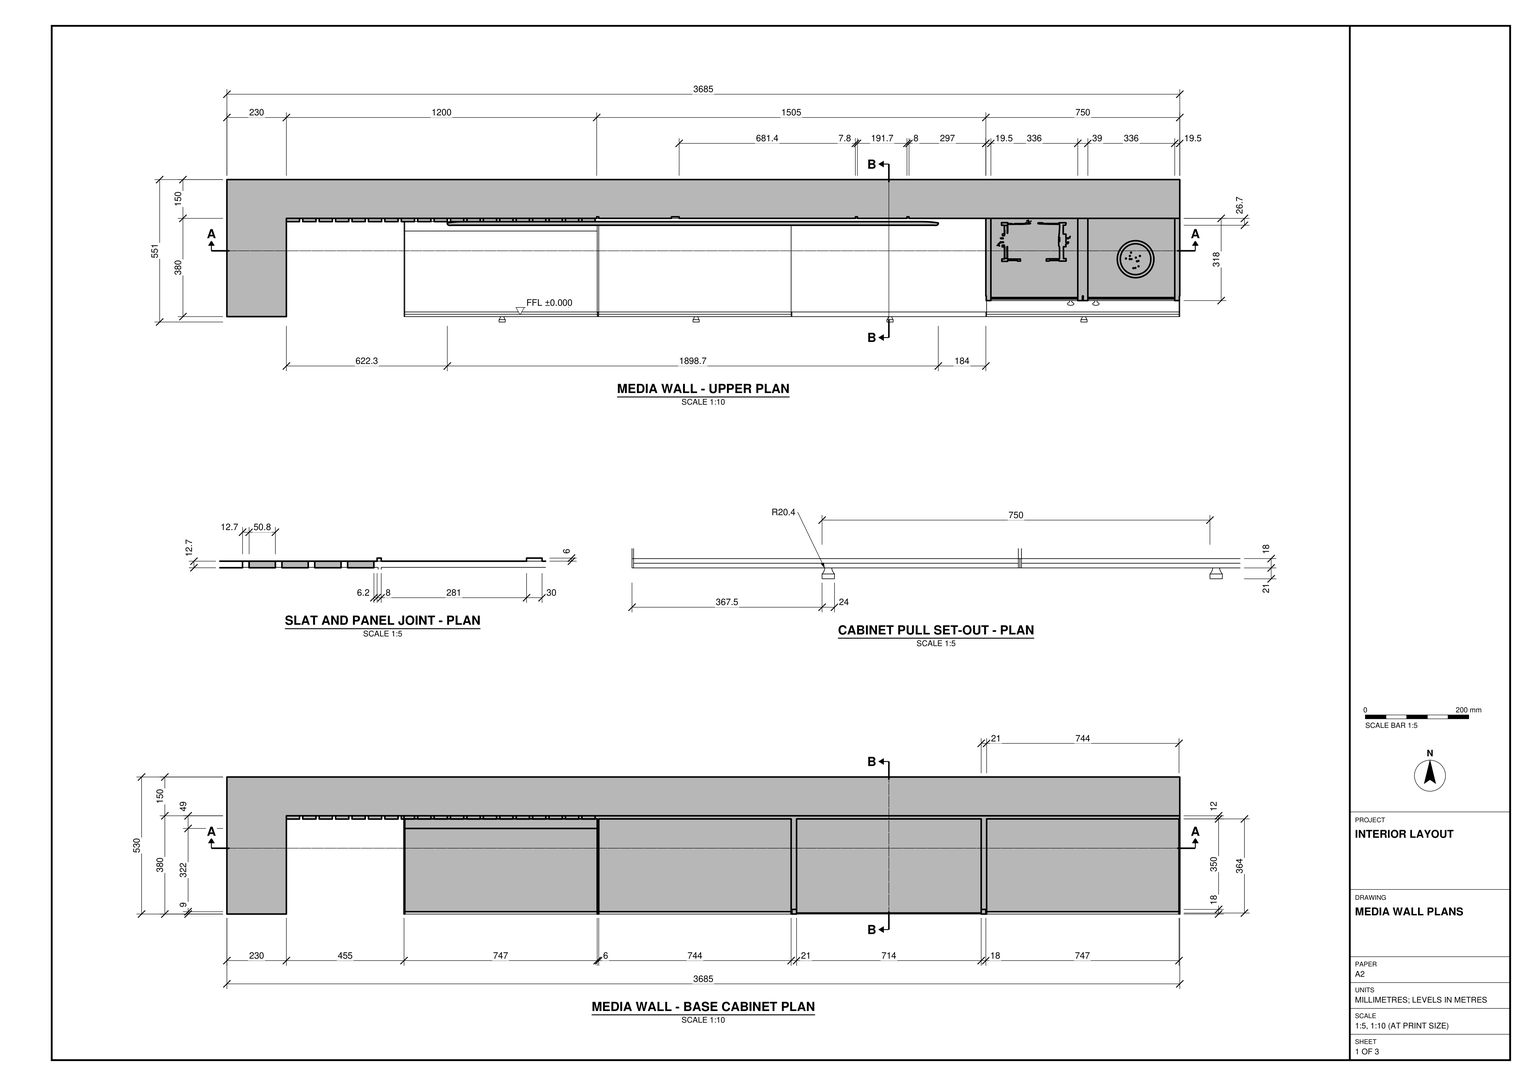
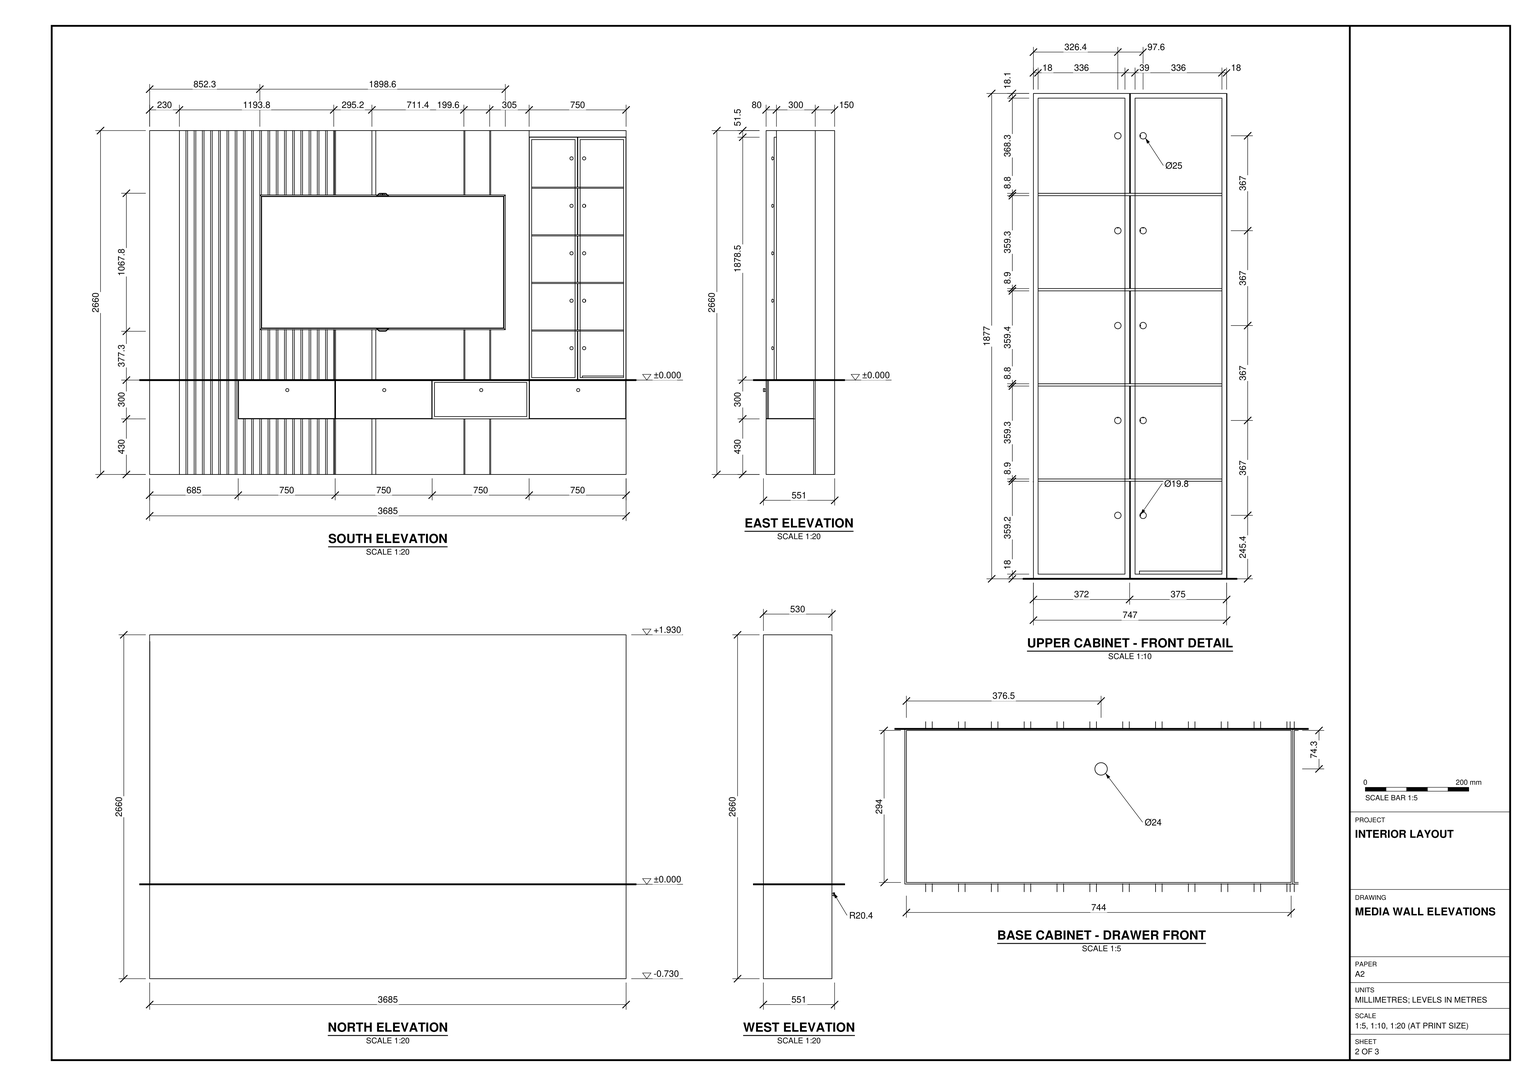
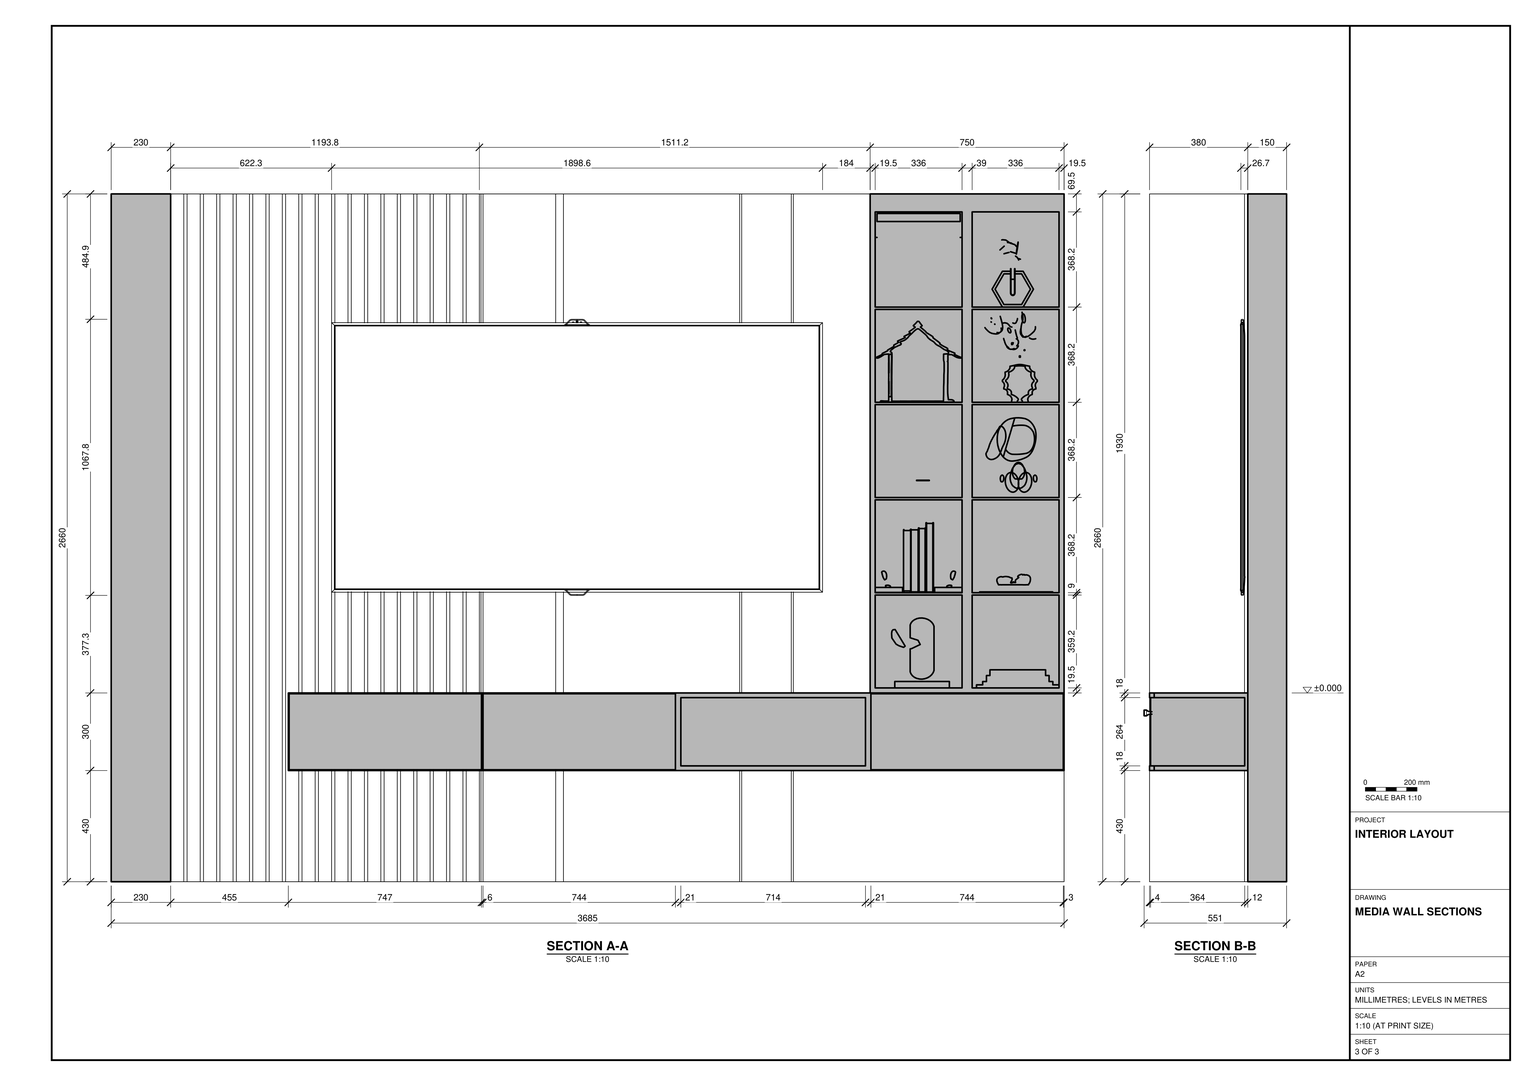
Build the media wall in SketchUp from task_files/diagram_01.pdf. Work in millimetres. The complete assembly, including the projecting cabinet pulls, is 3685 mm wide, 551 mm deep and 2660 mm high. Use the 0 mm datum shown at the top of the base cabinets: the wall extends from −730 mm to 1930 mm relative to that datum.

Use the plans to form the 150 mm thick backing wall and its left return. Facing the wall as in the south elevation, start the vertical slats immediately to the right of the return. Continue with flat panels, following the joint positions in the drawings. Place the screen across the transition from slats to panels. Below it, model the floating run of four base cabinet bays, including the drawer fronts, inset front detail and projecting pulls. Leave the wall face visible beneath the run.

At the right end, model the upper display cabinet with its centre divider, aligned shelves, framed fronts and pulls. Place books and loose display objects on the shelves as shown; any suitable library components may be used for these items. Keep the wall and each joinery piece in separate groups or components, and use components for repeated parts such as slats and pulls. Save one SketchUp model as output_files/media_wall_with_floating_cabinets_and_display_shelves.skp.

# SketchUp Ruby script. Lengths in millimetres.
U = 1.mm
M = Sketchup.active_model
def pt(a) = Geom::Point3d.new(a.map { |v| v * U })
def face(e, loops, mat)
  f = e.add_face(loops[0].map { |a| pt(a) })
  loops[1..].each { |l| e.add_face(l.map { |a| pt(a) }).erase! }
  f.material = f.back_material = mat if mat
  f
end
# faces: each face lists its corners as indices into pts; further lists are holes
def faces(e, pts, list, mat = nil) = list.each { |f| face(e, (f[0].is_a?(Array) ? f : [f]).map { |l| l.map { |i| pts[i] } }, mat) }
# xy, xz, yz: faces in a plane at the given z, y or x. An outline is a flat list of corners, or four numbers for a rectangle; further outlines are holes
def ring(l) = l.size == 4 ? [[l[0], l[1]], [l[2], l[1]], [l[2], l[3]], [l[0], l[3]]] : l.each_slice(2).to_a
def flat(e, list, mat, &to3) = list.each { |f| face(e, (f[0].is_a?(Array) ? f : [f]).map { |l| ring(l).map { |u, v| to3.(u, v) } }, mat) }
def xy(e, z, list, mat = nil) = flat(e, list, mat) { |x, y| [x, y, z] }
def xz(e, y, list, mat = nil) = flat(e, list, mat) { |x, z| [x, y, z] }
def yz(e, x, list, mat = nil) = flat(e, list, mat) { |y, z| [x, y, z] }
def lines(e, pts, list) = list.each { |a, b| e.add_line(pt(pts[a]), pt(pts[b])) }
# prism: a flat outline (further loops are holes) pulled along v
def prism(e, loops, v, mat = nil)
  f = face(e, loops, mat); d = Geom::Vector3d.new(v.map { |x| x * U })
  f.pushpull(f.normal.samedirection?(d) ? d.length : -d.length)
end
def box(e, o, s, mat = nil) = prism(e, [[o, [o[0] + s[0], o[1], o[2]], [o[0] + s[0], o[1] + s[1], o[2]], [o[0], o[1] + s[1], o[2]]]], [0, 0, s[2]], mat)
def at(x, y, z, deg = 0) = Geom::Transformation.translation(pt([x, y, z])) * Geom::Transformation.rotation(ORIGIN, Z_AXIS, deg.degrees)
def axes(o, x, y, z) = Geom::Transformation.new([*x, 0, *y, 0, *z, 0, *pt(o).to_a, 1])
def part(name) = M.definitions.add(name)
# library, detail: a bought-in or finely detailed component or shape, given as its bounding box
def library(name, o, s) = part(name).tap { |d| box(d.entities, o, s) }
def detail(e, o, s) = box(e.add_group.entities, o, s)
def put(e, d, t, mat = nil) = e.add_instance(d, t).tap { |i| i.material = mat if mat }
def group(e, t, mat = nil) = e.add_group.tap { |g| g.transformation = t; g.material = mat if mat }.entities
root = M.entities
M.materials.add("E04_Green_Bloom").color = [255, 255, 49]
M.materials.add("Plastic_Metalic_Black").color = [8, 8, 8]
M.materials.add("[Carpet Berber Multi]").color = [151, 134, 122]
M.materials.add("[Granite Dark Gray]").color = [69, 68, 68]
M.materials.add("[Metal Steel Textured]").color = [106, 110, 123]
M.materials.add("[Resin Turquoise]").color = [117, 218, 223]
M.materials.add("[Stone_Granite_Midnite]").color = [98, 95, 96]
M.materials.add("[Stone_Masonry_Multi]").color = [182, 175, 164]
M.materials.add("[Stone_Pavers_Flagstone_Gray]").color = [162, 162, 162]
M.materials.add("[Translucent Glass Blue]").color = [100, 149, 237]
M.materials["[Translucent Glass Blue]"].alpha = 0.5
M.materials.add("[Translucent Glass Dark Green]").color = [62, 91, 5]
M.materials["[Translucent Glass Dark Green]"].alpha = 0.5
M.materials.add("[Translucent Glass Tinted]").color = [8, 201, 241]
M.materials["[Translucent Glass Tinted]"].alpha = 0.5
M.materials.add("[Water Pool Light]").color = [64, 149, 167]
M.materials["[Water Pool Light]"].alpha = 0.6
M.materials.add("[Wood Bamboo]").color = [177, 105, 43]
M.materials.add("[Wood Floor Parquet]").color = [145, 89, 39]
M.materials.add("[Wood Veneer 01]").color = [120, 70, 37]
M.materials.add("[Wood Veneer 02]").color = [190, 128, 91]
c1 = part("Fluted wall panel")
box(c1.entities,[0,0,0],[50.8,12.7,2660])
box(c1.entities,[63.5,0,0],[50.8,12.7,2660])
box(c1.entities,[127,0,0],[50.8,12.7,2660])
box(c1.entities,[190.5,0,0],[50.8,12.7,2660])
box(c1.entities,[254,0,0],[50.8,12.7,2660])
box(c1.entities,[317.5,0,0],[50.8,12.7,2660])
box(c1.entities,[381,0,0],[50.8,12.7,2660])
box(c1.entities,[444.5,0,0],[50.8,12.7,2660])
box(c1.entities,[508,0,0],[50.8,12.7,2660])
box(c1.entities,[571.5,0,0],[50.8,12.7,2660])
box(c1.entities,[635,0,0],[50.8,12.7,2660])
box(c1.entities,[698.5,0,0],[50.8,12.7,2660])
box(c1.entities,[762,0,0],[50.8,12.7,2660])
box(c1.entities,[825.5,0,0],[50.8,12.7,2660])
box(c1.entities,[889,0,0],[50.8,12.7,2660])
box(c1.entities,[952.5,0,0],[50.8,12.7,2660])
box(c1.entities,[1016,0,0],[50.8,12.7,2660])
box(c1.entities,[1143,0,0],[50.8,12.7,2660])
xy(c1.entities,0,[[1079.5,0,1130.3,12.7]])
xy(c1.entities,2660,[[1079.5,0,1130.3,12.7]])
xz(c1.entities,0,[[1079.5,0,1130.3,2660]],"[Wood Floor Parquet]")
xz(c1.entities,12.7,[[1079.5,0,1130.3,2660]])
yz(c1.entities,1079.5,[[0,0,12.7,2660]])
yz(c1.entities,1130.3,[[0,0,12.7,2660]])
c2 = library("download?mid=50c7180b9fccec56d493bfe20f94b6ab&ctyp=sp&cv=p8.",[3795.5,1113.3,453.6],[1898.6,14.5,1067.8])
c3 = part("photo frame")
g1 = group(c3.entities,at(3094.9,8.6,0.8))
g2 = group(g1,at(0,0,0))
yz(g2,0,[[12.1,-0.8,0,0,33.6,534.4,45.7,533.6]],"Plastic_Metalic_Black")
yz(g2,8.6,[[7,8.2,39.5,525.3,33.1,525.8,0.5,8.6]],"Plastic_Metalic_Black")
yz(g2,393.2,[[7,8.2,0.5,8.6,33.1,525.8,39.5,525.3]],"Plastic_Metalic_Black")
yz(g2,401.8,[[12.1,-0.8,45.7,533.6,33.6,534.4,0,0]],"Plastic_Metalic_Black")
p = [[0,12.1,-0.8],[401.8,12.1,-0.8],[401.8,0,0],[0,0,0],[401.8,45.7,533.6],[0,45.7,533.6],
  [8.6,12.6,7.9],[393.2,12.6,7.9],[393.2,45.1,525],[8.6,45.1,525],[401.8,33.6,534.4],[0,33.6,534.4],
  [393.2,0.5,8.6],[8.6,0.5,8.6],[8.6,33.1,525.8],[393.2,33.1,525.8],[393.2,7,8.2],[8.6,7,8.2],
  [393.2,39.5,525.3],[8.6,39.5,525.3],[358.7,9.2,42.7],[43.2,9.2,42.7],[43.2,37.4,490.9],[358.7,37.4,490.9]]
faces(g2,p,[[0,1,2,3],[[4,1,0,5],[6,7,8,9]],[[2,10,11,3],[12,13,14,15]],[16,17,13,12],[19,18,15,14],[4,5,11,10]],"Plastic_Metalic_Black")
faces(g2,p,[[[17,16,18,19],[20,21,22,23]],[21,20,23,22]])
lines(g2,p,[[6,17],[9,19],[8,18],[7,16]])
c4 = library("Hexagonal flower vase",[-26.2,-52.8,0],[186.2,162.5,287.3])
c5 = library("Hexagonal flower vase \#1",[-6.8,-48.8,-5.9],[192.1,162.5,293.2])
c6 = library("Miniature+Toy+House+–+Teal+Roof,+Yellow+Trim,+and+Heart-Shap",[-518,0,0],[1389.1,735.6,998.2])
c7 = library("Copper+Vase+W.+Flowers",[-61.6,-66.4,0],[634.8,593.9,639.8])
c8 = library("Children's+Sailboat+Wall+Shelf++Decorative+Nursery+Bookcase+",[77.4,0,793.6],[1200,350,1226.4])
c9 = library("cheburashka",[1021,1096.6,-13.6],[484.8,208,352.2])
c10 = library("APARADOR+DE+LIVROS+CACHORRO",[2417,259.3,62.1],[359.3,219.7,270.8])
c11 = library("Buddha Fountain",[-19.2,-33.2,-3.3],[3019.4,1766,2624.3])
c12 = library("HORSE",[1857.3,-2493,-0.9],[2418.1,1518.6,2900.9])
c13 = library("16-POIGNEE CLC2",[-12.8,-12.5,0],[25,25,25])
c14 = library("14-POIGNEE CLC2",[-12,-12,0],[24,24,30])
c15 = library("Grupo\#181",[-9.6,-14,0],[182,201.9,289.1])
xy(root,0,[[0,0,230,530],[230,380,3685,530]])
xy(root,430,[[685,0,1435,18]])
xy(root,430,[[685,18,3685,380]],"[Carpet Berber Multi]")
xy(root,430,[[1435,0,2185,18],[2185,0,2935,18],[2935,0,3685,18]],"[Metal Steel Textured]")
xy(root,433,[[688,9,1432,18],[1438,9,2182,18],[2938,9,3682,18],[688,18,1432,368],[1438,18,2182,368],
  [2938,18,3682,368]],"[Carpet Berber Multi]")
xy(root,433,[[688,0,1432,9],[1438,0,2182,9],[2938,0,3682,9]],"[Metal Steel Textured]")
xy(root,448,[[2203,4,2917,18],[2203,18,2917,368]],"[Carpet Berber Multi]")
xy(root,448,[[2203,0,2917,4]],"[Metal Steel Textured]")
xy(root,712,[[2203,4,2917,18],[2203,18,2917,368]],"[Carpet Berber Multi]")
xy(root,712,[[2203,0,2917,4]],"[Metal Steel Textured]")
xy(root,727,[[688,9,1432,18],[1438,9,2182,18],[2938,9,3682,18],[688,18,1432,368],[1438,18,2182,368],
  [2938,18,3682,368]],"[Carpet Berber Multi]")
xy(root,727,[[688,0,1432,9],[1438,0,2182,9],[2938,0,3682,9]],"[Metal Steel Textured]")
xy(root,730,[[1430,380,1438,386],[1719,380,1749,386],[2430.4,380,2438.3,386],[2630,380,2638,386]])
xy(root,730,[[685,18,3685,18,3685,80,2935,80,2935,380,685,380]],"[Carpet Berber Multi]")
xy(root,730,[[685,0,1435,18],[1435,0,2185,18],[2185,0,2935,18],[2935,0,3685,18]],"[Metal Steel Textured]")
xy(root,730,[[2935,80,3685,380]],"[Wood Veneer 01]")
xy(root,731.5,[[2936.5,62,3308.5,80],[3308.5,62,3310,80],[3310,62,3311.5,80],[3311.5,62,3683.5,80]],"[Wood Veneer 01]")
xy(root,749.5,[[3346.4,68.5,3665.5,73.5]])
xy(root,749.5,[[2954.5,62,3290.5,68.5],[3329.5,62,3665.5,68.5]],"[Metal Steel Textured]")
xy(root,749.5,[[2954.5,68.5,3290.5,73.5],[3329.5,68.5,3346.4,73.5]],"[Translucent Glass Tinted]")
xy(root,749.5,[[2954.5,73.5,3290.5,380],[3329.5,73.5,3346.4,73.5,3346.4,331.9,3665.5,331.9,3665.5,380,3329.5,380],[3346.4,73.5,3665.5,331.9]],"[Wood Veneer 01]")
xy(root,761.4,[[[3346.4,73.5,3665.5,331.9],[3370.3,92.8,3641.6,301.1]]],"[Stone_Masonry_Multi]")
xy(root,774.1,[[[3370.3,92.8,3641.6,301.1],[3384.9,111.7,3627,282.3]]],"[Stone_Masonry_Multi]")
xy(root,797.4,[[[3384.9,111.7,3627,282.3],[3398.3,130,3613.6,264.9]]],"[Stone_Masonry_Multi]")
xy(root,819.6,[[[3398.3,130,3613.6,264.9],[3424.8,156.6,3598.4,238.2]]],"[Stone_Masonry_Multi]")
xy(root,926.4,[[3424.8,156.6,3598.4,238.2]],"[Stone_Pavers_Flagstone_Gray]")
xy(root,1108.7,[[2954.5,62,3290.5,80],[3290.5,62,3308.5,80],[3308.5,62,3310,80],[3310,62,3311.5,80],[3311.5,62,3329.5,80],
  [3329.5,62,3665.5,80],[2954.5,80,3290.5,380],[3329.5,80,3665.5,380]],"[Wood Veneer 01]")
xy(root,1117.5,[[2954.5,68.5,3290.5,73.5],[3329.5,68.5,3665.5,73.5]],"[Translucent Glass Tinted]")
xy(root,1117.7,[[2954.5,68.5,3290.5,73.5],[3329.5,68.5,3665.5,73.5]],"[Translucent Glass Tinted]")
xy(root,1117.7,[[2954.5,62,3290.5,68.5],[3290.5,62,3308.5,80],[3308.5,62,3310,80],[3310,62,3311.5,80],[3311.5,62,3329.5,80],
  [3329.5,62,3665.5,68.5],[2954.5,73.5,3290.5,380],[3329.5,73.5,3665.5,380]],"[Wood Veneer 01]")
xy(root,1476.9,[[2954.5,62,3290.5,380],[3290.5,62,3308.5,80],[3308.5,62,3310,80],[3310,62,3311.5,80],[3311.5,62,3329.5,80],
  [3329.5,62,3665.5,380]],"[Wood Veneer 01]")
xy(root,1485.7,[[2954.5,68.5,3290.5,73.5],[3329.5,68.5,3665.5,73.5]],"[Translucent Glass Tinted]")
xy(root,1485.9,[[2954.5,62,3290.5,68.5],[3329.5,62,3665.5,68.5]],"[Metal Steel Textured]")
xy(root,1485.9,[[2954.5,68.5,3290.5,73.5],[3329.5,68.5,3665.5,73.5]],"[Translucent Glass Tinted]")
xy(root,1485.9,[[3290.5,62,3308.5,80],[3308.5,62,3310,80],[3310,62,3311.5,80],[3311.5,62,3329.5,80],[2954.5,73.5,3290.5,380],
  [3329.5,73.5,3665.5,380]],"[Wood Veneer 01]")
xy(root,1845.1,[[2954.5,62,3290.5,380],[3290.5,62,3308.5,80],[3308.5,62,3310,80],[3310,62,3311.5,80],[3311.5,62,3329.5,80],
  [3329.5,62,3665.5,80],[3329.5,80,3665.5,380]],"[Wood Veneer 01]")
xy(root,1853.9,[[2954.5,68.5,3290.5,73.5],[3329.5,68.5,3665.5,73.5]],"[Translucent Glass Tinted]")
xy(root,1854.1,[[3329.5,62,3665.5,68.5]],"[Metal Steel Textured]")
xy(root,1854.1,[[2954.5,68.5,3290.5,73.5],[3329.5,68.5,3665.5,73.5]],"[Translucent Glass Tinted]")
xy(root,1854.1,[[2954.5,62,3290.5,68.5],[3290.5,62,3308.5,80],[3308.5,62,3310,80],[3310,62,3311.5,80],[3311.5,62,3329.5,80],
  [2954.5,73.5,3290.5,380],[3329.5,73.5,3665.5,380]],"[Wood Veneer 01]")
xy(root,2213.3,[[2954.5,62,3290.5,380],[3290.5,62,3308.5,80],[3308.5,62,3310,80],[3310,62,3311.5,80],[3311.5,62,3329.5,80],
  [3329.5,62,3665.5,380]],"[Wood Veneer 01]")
xy(root,2222.1,[[2954.5,68.5,3290.5,73.5],[3329.5,68.5,3665.5,73.5]],"[Translucent Glass Tinted]")
xy(root,2222.3,[[2954.5,62,3290.5,68.5],[3329.5,62,3665.5,68.5]],"[Metal Steel Textured]")
xy(root,2222.3,[[2954.5,68.5,3290.5,73.5],[3329.5,68.5,3665.5,73.5]],"[Translucent Glass Tinted]")
xy(root,2222.3,[[3290.5,62,3308.5,80],[3308.5,62,3310,80],[3310,62,3311.5,80],[3311.5,62,3329.5,80],[2954.5,73.5,3290.5,380],
  [3329.5,73.5,3665.5,380]],"[Wood Veneer 01]")
xy(root,2590.3,[[2954.5,68.5,3290.5,73.5],[3329.5,68.5,3665.5,73.5]],"[Translucent Glass Tinted]")
xy(root,2590.5,[[2954.5,62,3290.5,68.5],[3329.5,62,3665.5,68.5],[2954.5,68.5,3290.5,80],[3329.5,68.5,3665.5,80],[2954.5,80,3290.5,380],
  [3329.5,80,3665.5,380]],"[Wood Veneer 01]")
xy(root,2608.5,[[2936.5,62,3308.5,80],[3311.5,62,3683.5,80]],"[Metal Steel Textured]")
xy(root,2608.5,[[3308.5,62,3310,80],[3310,62,3311.5,80]],"[Wood Veneer 01]")
xy(root,2660,[[0,0,230,0,230,380,1430,380,1430,386,1438,386,1438,380,1719,380,1719,386,1749,386,1749,380,2430.4,380,2430.4,386,2438.3,386,2438.3,380,2630,380,2630,386,2638,386,2638,380,3685,380,3685,530,0,530]],"[Granite Dark Gray]")
xy(root,2660,[[2935,80,3685,380]],"[Wood Veneer 02]")
xz(root,0,[[0,0,230,2660]],"[Granite Dark Gray]")
xz(root,0,[[[685,430,1435,730],[688,433,1432,727]],[[1435,430,2185,730],[1438,433,2182,727]],[[2185,430,2935,730],[2203,448,2917,712]],[[2935,430,3685,730],[2938,433,3682,727]]],"[Metal Steel Textured]")
xz(root,4,[[2203,448,2917,712]],"[Translucent Glass Dark Green]")
xz(root,9,[[688,433,1432,727],[1438,433,2182,727],[2938,433,3682,727]],"[Translucent Glass Blue]")
xz(root,18,[[[685,430,1435,730],[688,433,1432,727]],[[1435,430,2185,730],[1438,433,2182,727]],[[2185,430,2935,730],[2203,448,2917,712]],[[2935,430,3685,730],[2938,433,3682,727]]])
xz(root,62,[[2936.5,731.5,3308.5,731.5,3308.5,1108.7,3290.5,1108.7,3290.5,749.5,2954.5,749.5,2954.5,2590.5,3290.5,2590.5,3290.5,2222.3,3308.5,2222.3,3308.5,2608.5,2936.5,2608.5],[3311.5,731.5,3683.5,731.5,3683.5,2608.5,3311.5,2608.5,3311.5,2222.3,3329.5,2222.3,3329.5,2590.5,3665.5,2590.5,3665.5,749.5,3329.5,749.5,3329.5,1108.7,3311.5,1108.7],[2954.5,1108.7,3665.5,1117.7],[3290.5,1117.7,3308.5,1476.9],[3311.5,1117.7,3329.5,1476.9],
  [2954.5,1476.9,3665.5,1485.9],[3290.5,1485.9,3308.5,1845.1],[3311.5,1485.9,3329.5,1845.1],[2954.5,1845.1,3665.5,1854.1],[3290.5,1854.1,3308.5,2213.3],
  [3311.5,1854.1,3329.5,2213.3],[2954.5,2213.3,3665.5,2222.3]],"[Metal Steel Textured]")
xz(root,62,[[3308.5,731.5,3310,1108.7],[3310,731.5,3311.5,1108.7],[3308.5,1117.7,3310,1476.9],[3310,1117.7,3311.5,1476.9],[3308.5,1485.9,3310,1845.1],
  [3310,1485.9,3311.5,1845.1],[3308.5,1854.1,3310,2213.3],[3310,1854.1,3311.5,2213.3],[3308.5,2222.3,3310,2608.5],[3310,2222.3,3311.5,2608.5]],"[Wood Veneer 01]")
xz(root,68.5,[[2954.5,749.5,3290.5,1117.5],[3329.5,749.5,3665.5,1117.5],[2954.5,1117.7,3290.5,1485.7],[3329.5,1117.7,3665.5,1485.7],[2954.5,1485.9,3290.5,1853.9],
  [3329.5,1485.9,3665.5,1853.9],[2954.5,1854.1,3290.5,2222.1],[3329.5,1854.1,3665.5,2222.1],[2954.5,2222.3,3290.5,2590.3],[3329.5,2222.3,3665.5,2590.3]],"[Translucent Glass Blue]")
xz(root,73.5,[[3346.4,749.5,3665.5,761.4]],"[Stone_Masonry_Multi]")
xz(root,73.5,[[2954.5,749.5,3290.5,1117.5],[3329.5,749.5,3329.5,1117.5,3665.5,1117.5,3665.5,761.4,3346.4,761.4,3346.4,749.5],[2954.5,1117.7,3290.5,1485.7],[3329.5,1117.7,3665.5,1485.7],[2954.5,1485.9,3290.5,1853.9],
  [3329.5,1485.9,3665.5,1853.9],[2954.5,1854.1,3290.5,2222.1],[3329.5,1854.1,3665.5,2222.1],[2954.5,2222.3,3290.5,2590.3],[3329.5,2222.3,3665.5,2590.3]],"[Translucent Glass Tinted]")
xz(root,80,[[[2935,730,3685,2610],[2936.5,731.5,3683.5,2608.5]],[3308.5,731.5,3310,1108.7],[3310,731.5,3311.5,1108.7],[3308.5,1117.7,3310,1476.9],[3310,1117.7,3311.5,1476.9],
  [3308.5,1485.9,3310,1845.1],[3310,1485.9,3311.5,1845.1],[3308.5,1854.1,3310,2213.3],[3310,1854.1,3311.5,2213.3],[3308.5,2222.3,3310,2608.5],
  [3310,2222.3,3311.5,2608.5]],"[Wood Veneer 01]")
xz(root,80,[[2935,2610,3685,2660]],"[Wood Veneer 02]")
xz(root,92.8,[[3370.3,761.4,3641.6,774.1]],"[Stone_Granite_Midnite]")
xz(root,111.7,[[3384.9,774.1,3627,797.4]],"[Stone_Granite_Midnite]")
xz(root,130,[[3398.3,797.4,3613.6,819.6]],"[Stone_Granite_Midnite]")
xz(root,156.6,[[3424.8,819.6,3598.4,926.4]],"[Stone_Pavers_Flagstone_Gray]")
xz(root,238.2,[[3424.8,819.6,3598.4,926.4]],"[Stone_Pavers_Flagstone_Gray]")
xz(root,264.9,[[3398.3,797.4,3613.6,819.6]],"[Stone_Granite_Midnite]")
xz(root,282.3,[[3384.9,774.1,3627,797.4]],"[Stone_Granite_Midnite]")
xz(root,301.1,[[3370.3,761.4,3641.6,774.1]],"[Stone_Granite_Midnite]")
xz(root,331.9,[[3346.4,749.5,3665.5,761.4]],"[Stone_Pavers_Flagstone_Gray]")
xz(root,368,[[688,433,1432,727]])
xz(root,368,[[1438,433,2182,727],[2938,433,3682,727],[2203,448,2917,712]],"[Carpet Berber Multi]")
xz(root,380,[[230,0,1430,0,1430,430,685,430,685,730,1430,730,1430,2660,230,2660],[1430,0,1438,430],[1438,0,1719,430],[1719,0,1749,430],[1749,0,2430.4,430],
  [2430.4,0,2438.3,430],[2438.3,0,2630,430],[2630,0,2638,430],[2638,0,3685,430],[1438,730,1719,2660],
  [1749,730,2430.4,2660],[2438.3,730,2630,2660],[2638,730,2935,2660]])
xz(root,380,[[2954.5,749.5,3290.5,1108.7],[3329.5,749.5,3665.5,1108.7],[2954.5,1126.7,3290.5,1476.9],[3329.5,1126.7,3665.5,1476.9],[3329.5,1494.9,3665.5,1845.1],
  [2954.5,1863.1,3290.5,2213.3],[3329.5,1863.1,3665.5,2213.3],[2954.5,2231.3,3290.5,2590.5],[3329.5,2231.3,3665.5,2590.5]],"[Water Pool Light]")
xz(root,380,[[685,430,1430,730],[1430,430,1438,730],[1438,430,1719,730],[1719,430,1749,730],[1749,430,2430.4,730],
  [2430.4,430,2438.3,730],[2438.3,430,2630,730],[2630,430,2638,730],[2638,430,3685,730],[[2935,730,3685,2660],[2954.5,2222.3,3290.5,2590.5],[3329.5,2222.3,3665.5,2590.5],[2954.5,1117.7,3290.5,1476.9],[3329.5,1117.7,3665.5,1476.9],[2954.5,1854.1,3290.5,2213.3],[3329.5,1854.1,3665.5,2213.3],[2954.5,749.5,3290.5,1108.7],[3329.5,749.5,3665.5,1108.7],[3329.5,1485.9,3665.5,1845.1],[2954.5,1485.9,3290.5,1845.1]],
  [2954.5,1117.7,3290.5,1126.7],[3329.5,1117.7,3665.5,1126.7],[2954.5,1485.9,3290.5,1494.9],[3329.5,1485.9,3665.5,1494.9],[2954.5,1494.9,3290.5,1845.1],
  [2954.5,1854.1,3290.5,1863.1],[3329.5,1854.1,3665.5,1863.1],[2954.5,2222.3,3290.5,2231.3],[3329.5,2222.3,3665.5,2231.3]],"[Wood Veneer 01]")
xz(root,386,[[1430,730,1438,2660],[1719,730,1749,2660],[2430.4,730,2438.3,2660],[2630,730,2638,2660]])
xz(root,530,[[0,0,3685,2660]])
yz(root,0,[[0,0,530,2660]],"[Granite Dark Gray]")
yz(root,230,[[0,0,380,2660]],"[Granite Dark Gray]")
yz(root,685,[[18,430,380,730]],"[Carpet Berber Multi]")
yz(root,685,[[0,430,18,730]],"[Metal Steel Textured]")
yz(root,688,[[9,433,18,727],[18,433,368,727]],"[Carpet Berber Multi]")
yz(root,688,[[0,433,9,727]],"[Metal Steel Textured]")
yz(root,1430,[[380,730,386,2660]])
yz(root,1432,[[9,433,18,727],[18,433,368,727]],"[Carpet Berber Multi]")
yz(root,1432,[[0,433,9,727]],"[Metal Steel Textured]")
yz(root,1435,[[0,430,18,730]])
yz(root,1438,[[380,730,386,2660]])
yz(root,1438,[[9,433,18,727],[18,433,368,727]],"[Carpet Berber Multi]")
yz(root,1438,[[0,433,9,727]],"[Metal Steel Textured]")
yz(root,1719,[[380,730,386,2660]])
yz(root,1749,[[380,730,386,2660]])
yz(root,2182,[[9,433,18,727],[18,433,368,727]],"[Carpet Berber Multi]")
yz(root,2182,[[0,433,9,727]],"[Metal Steel Textured]")
yz(root,2185,[[0,430,18,730]])
yz(root,2203,[[4,448,18,712],[18,448,368,712]],"[Carpet Berber Multi]")
yz(root,2203,[[0,448,4,712]],"[Metal Steel Textured]")
yz(root,2430.4,[[380,730,386,2660]])
yz(root,2438.3,[[380,730,386,2660]])
yz(root,2630,[[380,730,386,2660]])
yz(root,2638,[[380,730,386,2660]])
yz(root,2917,[[4,448,18,712],[18,448,368,712]],"[Carpet Berber Multi]")
yz(root,2917,[[0,448,4,712]],"[Metal Steel Textured]")
yz(root,2935,[[0,430,18,730]])
yz(root,2935,[[80,730,380,2610],[80,2610,380,2660]],"[Wood Veneer 02]")
yz(root,2936.5,[[62,731.5,80,2608.5]],"[Metal Steel Textured]")
yz(root,2938,[[9,433,18,727],[18,433,368,727]],"[Carpet Berber Multi]")
yz(root,2938,[[0,433,9,727]],"[Metal Steel Textured]")
yz(root,2954.5,[[62,749.5,68.5,1108.7]],"[Metal Steel Textured]")
yz(root,2954.5,[[68.5,749.5,73.5,1108.7],[68.5,1117.7,73.5,1476.9],[68.5,1485.9,73.5,1845.1],[68.5,1854.1,73.5,2213.3],[68.5,2222.3,73.5,2590.3]],"[Translucent Glass Tinted]")
yz(root,2954.5,[[73.5,749.5,380,1108.7],[62,1108.7,68.5,1117.7],[68.5,1108.7,73.5,1117.5],[73.5,1108.7,80,1108.7,80,1117.7,68.5,1117.7,68.5,1117.5,73.5,1117.5],[62,1117.7,68.5,1476.9],
  [73.5,1117.7,380,1476.9],[62,1476.9,68.5,1485.9],[68.5,1476.9,73.5,1485.7],[73.5,1476.9,80,1476.9,80,1485.9,68.5,1485.9,68.5,1485.7,73.5,1485.7],[62,1485.9,68.5,1845.1],
  [73.5,1485.9,380,1845.1],[62,1845.1,68.5,1854.1],[68.5,1845.1,73.5,1853.9],[73.5,1845.1,80,1845.1,80,1854.1,68.5,1854.1,68.5,1853.9,73.5,1853.9],[62,1854.1,68.5,2213.3],
  [73.5,1854.1,380,2213.3],[62,2213.3,68.5,2222.3],[68.5,2213.3,73.5,2222.1],[73.5,2213.3,80,2213.3,80,2222.3,68.5,2222.3,68.5,2222.1,73.5,2222.1],[62,2222.3,68.5,2222.3,68.5,2590.3,73.5,2590.3,73.5,2222.3,380,2222.3,380,2590.5,62,2590.5]],"[Wood Veneer 01]")
yz(root,3290.5,[[62,749.5,68.5,1108.7],[62,1117.7,68.5,1476.9],[62,1485.9,68.5,1845.1],[62,1854.1,68.5,2213.3]],"[Metal Steel Textured]")
yz(root,3290.5,[[68.5,1108.7,73.5,1117.5],[68.5,1476.9,73.5,1485.7],[68.5,1845.1,73.5,1853.9],[68.5,2213.3,73.5,2222.1],[68.5,2222.3,73.5,2590.3]],"[Translucent Glass Tinted]")
yz(root,3290.5,[[68.5,749.5,73.5,1108.7],[73.5,749.5,380,1108.7],[68.5,1117.7,73.5,1476.9],[73.5,1117.7,380,1476.9],[68.5,1485.9,73.5,1845.1],
  [73.5,1485.9,380,1845.1],[68.5,1854.1,73.5,2213.3],[73.5,1854.1,380,2213.3],[62,2222.3,62,2590.5,380,2590.5,380,2222.3,73.5,2222.3,73.5,2590.3,68.5,2590.3,68.5,2222.3]],"[Wood Veneer 01]")
yz(root,3308.5,[[62,731.5,80,1108.7],[62,1117.7,80,1476.9],[62,1485.9,80,1845.1],[62,1854.1,80,2213.3],[62,2222.3,80,2608.5]],"[Wood Veneer 01]")
yz(root,3310,[[62,731.5,80,1108.7],[62,1117.7,80,1476.9],[62,1485.9,80,1845.1],[62,1854.1,80,2213.3],[62,2222.3,80,2608.5]],"[Wood Veneer 01]")
yz(root,3311.5,[[62,731.5,80,1108.7],[62,1117.7,80,1476.9],[62,1485.9,80,1845.1],[62,1854.1,80,2213.3],[62,2222.3,80,2608.5]],"[Wood Veneer 01]")
yz(root,3329.5,[[62,749.5,68.5,1108.7]],"[Metal Steel Textured]")
yz(root,3329.5,[[68.5,749.5,73.5,1108.7],[68.5,1117.7,73.5,1476.9],[68.5,1485.9,73.5,1845.1],[68.5,1854.1,73.5,2213.3],[68.5,2213.3,73.5,2222.1],
  [68.5,2222.3,73.5,2590.3]],"[Translucent Glass Tinted]")
yz(root,3329.5,[[73.5,749.5,380,1108.7],[62,1117.7,68.5,1476.9],[73.5,1117.7,380,1476.9],[62,1485.9,68.5,1845.1],[73.5,1485.9,380,1845.1],
  [62,1854.1,68.5,2213.3],[73.5,1854.1,380,2213.3],[62,2222.3,68.5,2222.3,68.5,2590.3,73.5,2590.3,73.5,2222.3,380,2222.3,380,2590.5,62,2590.5]],"[Wood Veneer 01]")
yz(root,3346.4,[[73.5,749.5,331.9,761.4]],"[Stone_Pavers_Flagstone_Gray]")
yz(root,3370.3,[[92.8,761.4,301.1,774.1]],"[Stone_Pavers_Flagstone_Gray]")
yz(root,3384.9,[[111.7,774.1,282.3,797.4]],"[Stone_Granite_Midnite]")
yz(root,3398.3,[[130,797.4,264.9,819.6]],"[Stone_Granite_Midnite]")
yz(root,3424.8,[[156.6,819.6,238.2,926.4]],"[Stone_Pavers_Flagstone_Gray]")
yz(root,3598.4,[[156.6,819.6,238.2,926.4]],"[Stone_Pavers_Flagstone_Gray]")
yz(root,3613.6,[[130,797.4,264.9,819.6]],"[Stone_Granite_Midnite]")
yz(root,3627,[[111.7,774.1,282.3,797.4]],"[Stone_Granite_Midnite]")
yz(root,3641.6,[[92.8,761.4,301.1,774.1]],"[Stone_Granite_Midnite]")
yz(root,3665.5,[[62,761.4,68.5,1108.7],[62,1117.7,68.5,1476.9],[62,1485.9,68.5,1845.1],[62,1854.1,68.5,2213.3]],"[Metal Steel Textured]")
yz(root,3665.5,[[62,749.5,68.5,761.4]],"[Stone_Pavers_Flagstone_Gray]")
yz(root,3665.5,[[68.5,1108.7,73.5,1117.5],[68.5,1476.9,73.5,1485.7],[68.5,1845.1,73.5,1853.9],[68.5,2213.3,73.5,2222.1],[68.5,2222.3,73.5,2590.3]],"[Translucent Glass Tinted]")
yz(root,3665.5,[[68.5,749.5,73.5,761.4],[331.9,749.5,331.9,761.4,73.5,761.4,73.5,1108.7,380,1108.7,380,749.5],[73.5,749.5,331.9,761.4],[68.5,761.4,73.5,1108.7],[62,1108.7,68.5,1117.7],
  [73.5,1108.7,73.5,1117.5,68.5,1117.5,68.5,1117.7,80,1117.7,80,1108.7],[68.5,1117.7,73.5,1476.9],[73.5,1117.7,380,1476.9],[62,1476.9,68.5,1485.9],[73.5,1476.9,73.5,1485.7,68.5,1485.7,68.5,1485.9,80,1485.9,80,1476.9],
  [68.5,1485.9,73.5,1845.1],[73.5,1485.9,380,1845.1],[62,1845.1,68.5,1854.1],[73.5,1845.1,73.5,1853.9,68.5,1853.9,68.5,1854.1,80,1854.1,80,1845.1],[68.5,1854.1,73.5,2213.3],
  [73.5,1854.1,380,2213.3],[62,2213.3,68.5,2222.3],[73.5,2213.3,73.5,2222.1,68.5,2222.1,68.5,2222.3,80,2222.3,80,2213.3],[62,2222.3,62,2590.5,380,2590.5,380,2222.3,73.5,2222.3,73.5,2590.3,68.5,2590.3,68.5,2222.3]],"[Wood Veneer 01]")
yz(root,3682,[[9,433,18,727],[18,433,368,727]],"[Carpet Berber Multi]")
yz(root,3682,[[0,433,9,727]],"[Metal Steel Textured]")
yz(root,3683.5,[[62,731.5,80,2608.5]],"[Metal Steel Textured]")
yz(root,3685,[[380,0,530,2660]],"[Granite Dark Gray]")
yz(root,3685,[[0,430,18,730]],"[Metal Steel Textured]")
yz(root,3685,[[18,430,380,730]],"[Wood Veneer 01]")
yz(root,3685,[[80,730,380,2660]],"[Wood Veneer 02]")
p = [[2936.5,380,1106.9],[2935,380,1106.9],[3671.2,71,2575.3],[3671.2,71,2207.1],[3290.5,68.5,2222.3],[3290.5,68.5,2222.1],
  [3290.5,68.5,1854.1],[3290.5,68.5,1853.9],[3290.5,68.5,1485.9],[3290.5,68.5,1485.7],[3290.5,68.5,1117.7],[3290.5,68.5,1117.5],
  [3329.5,68.5,2222.1],[3329.5,68.5,2222.3],[3329.5,68.5,1853.9],[3329.5,68.5,1854.1],[3329.5,68.5,1117.5],[3329.5,68.5,1117.7],
  [3329.5,68.5,1485.7],[3329.5,68.5,1485.9],[3370.3,301.1,749.5],[3370.3,92.8,749.5],[3641.6,92.8,749.5],[3641.6,301.1,749.5],
  [3370.3,92.8,761.4],[3370.3,301.1,761.4],[3641.6,92.8,761.4],[3641.6,301.1,761.4]]
lines(root,p,[[0,1],[2,3],[4,5],[6,7],[8,9],[10,11],[12,13],[14,15],[16,17],[18,19],[20,21],[21,22],
  [22,23],[23,20],[21,24],[20,25],[22,26],[23,27]])
put(root,c1,at(230,367.3,0),"[Wood Bamboo]")
put(root,c2,at(-2943.2,-760.5,653.7))
put(root,c3,axes([366.7,208.6,2222.3],[0.83616,0,0],[0,1.01502,0],[0,0,0.68805]))
put(root,c4,at(3406.5,207.9,2222.3))
put(root,c5,axes([3541.5,180.6,2222.3],[0.5456,-0.315,0],[0.315,0.5456,0],[0,0,0.63]))
put(root,c6,axes([2954.5,265.4,1854.1],[0,-0.2138,0],[0.45679,0,0],[0,0,0.36633]))
put(root,c7,axes([3362.1,97.5,1854.1],[0.52935,0,0],[0,0.53545,0],[0,0,0.56146]))
put(root,c8,axes([3111.3,236.8,1473.3],[0.04102,0,0],[0,0.40921,0],[0,0,0.07791]))
put(root,c9,axes([2580.7,-924.6,1499.5],[0.73337,0,0],[0,1,0],[0,0,1]))
put(root,c10,axes([694,-99,1055.6],[0.93523,0,0],[0,1,0],[0,0,1]))
put(root,c11,axes([3331.6,68,1118.1],[0.11128,0,0],[0,0.18007,0],[0,0,0.13688]),"[Water Pool Light]")
put(root,c12,axes([3405.3,273.5,928.2],[0.03706,0,0],[0,0.0478,0],[0,0,0.06225]),"E04_Green_Bloom")
put(root,c13,axes([3263.2,68.5,976.9],[1,0,0],[0,0,1],[0,-1,0]))
put(root,c13,axes([3263.2,68.5,1343.9],[1,0,0],[0,0,1],[0,-1,0]))
put(root,c13,axes([3263.2,68.5,1710.9],[1,0,0],[0,0,1],[0,-1,0]))
put(root,c13,axes([3263.2,68.5,2077.9],[1,0,0],[0,0,1],[0,-1,0]))
put(root,c13,axes([3263.2,68.5,2444.9],[1,0,0],[0,0,1],[0,-1,0]),"[Resin Turquoise]")
put(root,c13,axes([3360.9,68.5,2077.9],[1,0,0],[0,0,1],[0,-1,0]))
put(root,c13,axes([3360.9,68.5,1710.9],[1,0,0],[0,0,1],[0,-1,0]))
put(root,c13,axes([3360.9,68.5,1343.9],[1,0,0],[0,0,1],[0,-1,0]))
put(root,c13,axes([3360.9,68.5,2444.9],[1,0,0],[0,0,1],[0,-1,0]))
put(root,c13,axes([3360.9,68.5,976.9],[1,0,0],[0,0,1],[0,-1,0]))
put(root,c14,axes([1064.5,9,652.7],[1,0,0],[0,0,1],[0,-1,0]))
put(root,c14,axes([1814.5,9,652.7],[1,0,0],[0,0,1],[0,-1,0]))
put(root,c14,axes([2564.5,9,652.7],[1,0,0],[0,0,1],[0,-1,0]))
put(root,c14,axes([3314.5,9,652.7],[1,0,0],[0,0,1],[0,-1,0]))
g3 = group(root,at(688,331,433),"[Carpet Berber Multi]")
xz(g3,0,[[0,0,744,294]])
put(root,c15,axes([2983.9,195.4,749.5],[1.83826,0.11565,0],[-0.06218,0.98831,0],[0,0,1.24235]))
